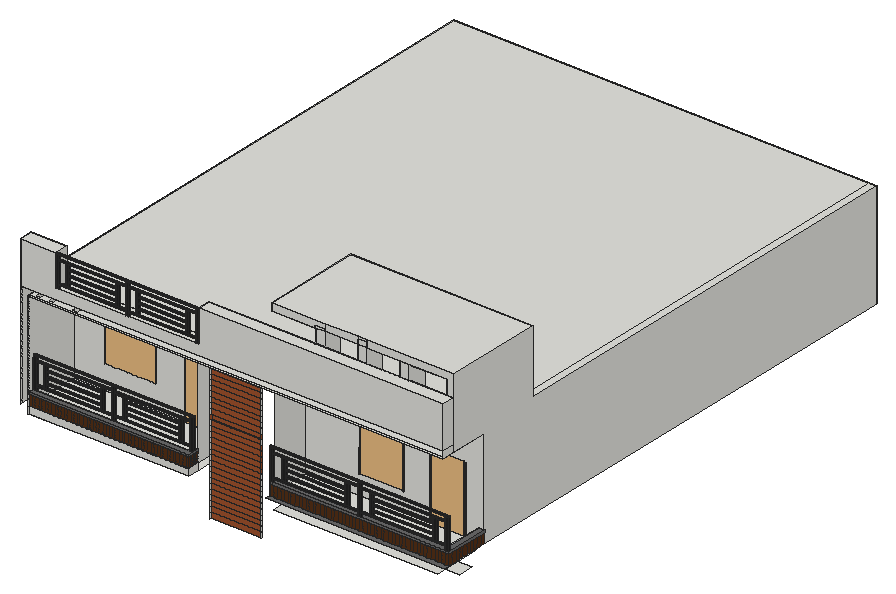
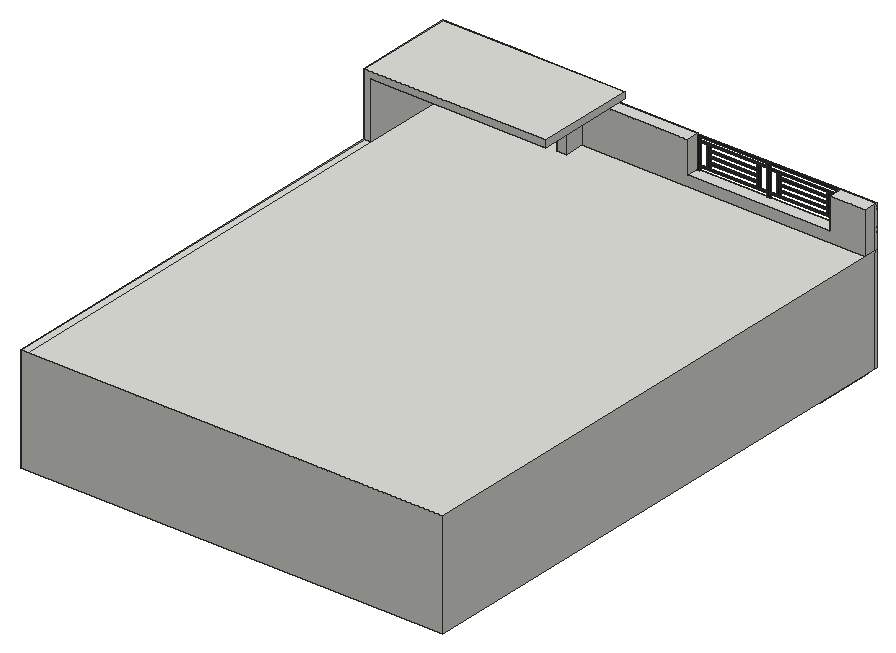
# SketchUp Ruby script. Lengths in inches.
U = 1.inch
M = Sketchup.active_model
def pt(a) = Geom::Point3d.new(a.map { |v| v * U })
def face(e, loops, mat)
  f = e.add_face(loops[0].map { |a| pt(a) })
  loops[1..].each { |l| e.add_face(l.map { |a| pt(a) }).erase! }
  f.material = f.back_material = mat if mat
  f
end
# faces: each face lists its corners as indices into pts; further lists are holes
def faces(e, pts, list, mat = nil) = list.each { |f| face(e, (f[0].is_a?(Array) ? f : [f]).map { |l| l.map { |i| pts[i] } }, mat) }
# xy, xz, yz: faces in a plane at the given z, y or x. An outline is a flat list of corners, or four numbers for a rectangle; further outlines are holes
def ring(l) = l.size == 4 ? [[l[0], l[1]], [l[2], l[1]], [l[2], l[3]], [l[0], l[3]]] : l.each_slice(2).to_a
def flat(e, list, mat, &to3) = list.each { |f| face(e, (f[0].is_a?(Array) ? f : [f]).map { |l| ring(l).map { |u, v| to3.(u, v) } }, mat) }
def xy(e, z, list, mat = nil) = flat(e, list, mat) { |x, y| [x, y, z] }
def xz(e, y, list, mat = nil) = flat(e, list, mat) { |x, z| [x, y, z] }
def yz(e, x, list, mat = nil) = flat(e, list, mat) { |y, z| [x, y, z] }
def lines(e, pts, list) = list.each { |a, b| e.add_line(pt(pts[a]), pt(pts[b])) }
# prism: a flat outline (further loops are holes) pulled along v
def prism(e, loops, v, mat = nil)
  f = face(e, loops, mat); d = Geom::Vector3d.new(v.map { |x| x * U })
  f.pushpull(f.normal.samedirection?(d) ? d.length : -d.length)
end
def box(e, o, s, mat = nil) = prism(e, [[o, [o[0] + s[0], o[1], o[2]], [o[0] + s[0], o[1] + s[1], o[2]], [o[0], o[1] + s[1], o[2]]]], [0, 0, s[2]], mat)
def at(x, y, z, deg = 0) = Geom::Transformation.translation(pt([x, y, z])) * Geom::Transformation.rotation(ORIGIN, Z_AXIS, deg.degrees)
def axes(o, x, y, z) = Geom::Transformation.new([*x, 0, *y, 0, *z, 0, *pt(o).to_a, 1])
def part(name) = M.definitions.add(name)
# library, detail: a bought-in or finely detailed component or shape, given as its bounding box
def library(name, o, s) = part(name).tap { |d| box(d.entities, o, s) }
def detail(e, o, s) = box(e.add_group.entities, o, s)
def put(e, d, t, mat = nil) = e.add_instance(d, t).tap { |i| i.material = mat if mat }
def group(e, t, mat = nil) = e.add_group.tap { |g| g.transformation = t; g.material = mat if mat }.entities
root = M.entities
M.materials.add("Painted Metal Railing").color = [35, 35, 35]
M.materials.add("[0042_Sienna]").color = [160, 82, 45]
M.materials.add("[0134_DimGray]").color = [105, 105, 105]
M.materials.add("[Wood Cherry Original]").color = [86, 49, 23]
c1 = library("PINTU 6 YA",[0,-0.6875,0],[35.83,8.07,80.71])
c2 = part("Post")
box(c2.entities,[-0.75,-0.75,0],[1.5,1.5,34.5],"Painted Metal Railing")
c3 = part("Group43\#1")
box(c3.entities,[-0.75,0,0],[1.5,73.5,1.5],"Painted Metal Railing")
c4 = part("Group46\#2")
box(c4.entities,[-0.75,0.75,0],[1.5,34.5,1.5],"Painted Metal Railing")
c5 = part("Group49\#1")
box(c5.entities,[-0.75,0.75,0],[1.5,34.5,1.5],"Painted Metal Railing")
c6 = part("Group52\#1")
box(c6.entities,[-0.75,0.75,0],[1.5,34.5,1.5],"Painted Metal Railing")
c7 = part("Group55\#1")
box(c7.entities,[-0.75,0.75,0],[1.5,34.5,1.5],"Painted Metal Railing")
c8 = part("Inner Post")
box(c8.entities,[-0.75,-0.75,0],[1.5,1.5,23.5],"Painted Metal Railing")
c9 = part("Group59\#1")
box(c9.entities,[-0.75,0.75,0],[1.5,24.5,1.5],"Painted Metal Railing")
c10 = part("Group62\#1")
box(c10.entities,[-0.75,0.75,0],[1.5,24.5,1.5],"Painted Metal Railing")
c11 = part("Group65\#1")
box(c11.entities,[-0.75,0.75,0],[1.5,24.5,1.5],"Painted Metal Railing")
c12 = part("Inner Posts and Rails\#2")
put(c12.entities,c8,at(0,0,0,90))
put(c12.entities,c8,at(0,26,0,90))
put(c12.entities,c9,at(0,0,4.75))
put(c12.entities,c10,at(0,0,11))
put(c12.entities,c11,at(0,0,17.25))
c13 = part("Group69\#1")
box(c13.entities,[-0.75,0.75,0],[1.5,24.5,1.5],"Painted Metal Railing")
c14 = part("Group72\#1")
box(c14.entities,[-0.75,0.75,0],[1.5,24.5,1.5],"Painted Metal Railing")
c15 = part("Group75\#1")
box(c15.entities,[-0.75,0.75,0],[1.5,24.5,1.5],"Painted Metal Railing")
c16 = part("Inner Posts and Rails\#3")
put(c16.entities,c8,at(0,0,0,90))
put(c16.entities,c8,at(0,26,0,90))
put(c16.entities,c13,at(0,0,4.75))
put(c16.entities,c14,at(0,0,11))
put(c16.entities,c15,at(0,0,17.25))
c17 = part("Railing Assembly 14\#1")
put(c17.entities,c2,at(0,0,0))
put(c17.entities,c2,at(36,0,0))
put(c17.entities,c2,at(72,0,0))
put(c17.entities,c3,at(-0.75,0,34.5,-90))
put(c17.entities,c4,at(0,0,4,-90))
put(c17.entities,c5,at(36,0,4,-90))
put(c17.entities,c6,at(0,0,29,-90))
put(c17.entities,c7,at(36,0,29,-90))
put(c17.entities,c12,at(5,0,5.5,-90))
put(c17.entities,c16,at(41,0,5.5,-90))
c18 = library("Group\#6",[0,0,0],[8.07,62.0625,54])
xy(root,321.9375,[[415.76,55.8125,455.32,73]])
xy(root,323.32,[[334.19,55.8125,396.26,70.4375]])
xy(root,332.51,[[33.6,70.1875,103.97,80.1875]])
xy(root,335.1875,[[131.125,70.1875,180.3125,90.9375]])
xy(root,352,[[8,2.66,8,70.1875,189.625,70.1875,189.625,15.9375,190.03,15.9375,190.03,2.66],[286.5625,3.0625,472.04,55.8125]])
xy(root,360,[[8,2.66,190.03,2.66,190.03,15.9375,189.625,15.9375,189.625,3.0625,8,3.0625],[8,3.0625,8,9.0625,183.625,9.0625,183.625,15.9375,189.625,15.9375,189.625,3.0625],[8,9.0625,183.625,9.0625,183.625,15.9375,189.625,15.9375,189.625,66.3125,182.5,66.3125,182.5,77.1875,134.19,77.1875,134.19,66.3125,8,66.3125],[276.8125,9.0625,276.8125,15.9375,474,15.9375,474,59.375,480,59.375,480,9.0625],[276.8125,15.9375,474,15.9375,474,59.375,457.04,59.375,457.04,75.5,418.72,75.5,418.72,59.375,276.8125,59.375]])
xy(root,360,[[276.8125,3.0625,480,9.0625]],"[0134_DimGray]")
xy(root,372,[[8,2.66,190.03,3.0625],[8,3.0625,8,9.0625,183.625,9.0625,183.625,15.9375,189.625,15.9375,189.625,3.0625],[189.625,3.0625,190.03,15.9375],[276.8125,8.66,480.4,9.0625],[276.8125,9.0625,276.8125,15.9375,474,15.9375,474,59.375,480,59.375,480,9.0625],
  [480,9.0625,480.4,59.375]])
xy(root,374,[[8,2.66,190.03,2.66,190.03,15.9375,183.625,15.9375,183.625,9.0625,8,9.0625]],"[0134_DimGray]")
xy(root,374.875,[[276.8125,8.66,480.4,8.66,480.4,59.375,474,59.375,474,15.9375,276.8125,15.9375]],"[0134_DimGray]")
xy(root,381.34,[[338.1875,59.375,387.9375,69.0625]])
xy(root,387.125,[[44.07,66.3125,101.07,89.625]])
xy(root,407.98,[[203.35,17.0625,260.98,18.1875]],"[0042_Sienna]")
xy(root,413.85,[[203.35,17.0625,260.98,18.1875]])
xy(root,436.06,[[338.28,59.375,388.03,69.0625]])
xy(root,436.3125,[[418.72,59.375,457.04,75.5]])
xy(root,440.4375,[[44.07,66.3125,101.07,89.625]])
xy(root,446.5625,[[134.19,66.3125,182.5,77.1875]])
xy(root,460.87,[[203.35,15.54,260.98,17.0625]])
xy(root,466.75,[[203.35,15.54,260.98,17.0625]],"[0042_Sienna]")
xy(root,471.9375,[[41.12,5.07,47.93,11.88]])
xy(root,472.625,[[8,1,480,3.0625],[[8,3.0625,8,66.3125,189.625,66.3125,189.625,15.9375,203.35,15.9375,203.35,17.0625,260.98,17.0625,260.98,15.9375,276.8125,15.9375,276.8125,59.375,480,59.375,480,3.0625],[13.71,5.07,20.52,11.88],[27.41,5.07,34.23,11.88],[54.83,5.07,61.64,11.88]]])
xy(root,480,[[0,1,480,15.9375],[0,15.9375,322.54,15.9375,322.54,37.75,333.36,37.75,333.36,15.9375,370.7,15.9375,370.7,37.75,381.51,37.75,381.51,15.9375,418.86,15.9375,418.86,37.75,429.67,37.75,429.67,15.9375,472,15.9375,472,615.9375,0,615.9375],[472,128.18,480,615.9375]])
xy(root,491.72,[[40.47,1,202.15,15.9375]])
xy(root,528,[[0,1,40.47,15.9375],[202.15,1,480,15.9375],[322.54,15.9375,333.36,17.25]])
xy(root,544,[[273.3125,15.9375,273.3125,128.18,472,128.18,472,15.9375,429.67,15.9375,429.67,37.75,418.86,37.75,418.86,15.9375,333.36,15.9375,333.36,17.25,322.54,17.25,322.54,15.9375],[322.54,15.9375,333.36,17.25]])
xy(root,546.3125,[[322.54,15.9375,333.36,37.75]])
xy(root,549.9375,[[370.7,15.9375,381.51,37.75]])
xy(root,552,[[273.3125,15.9375,480,128.18]])
xz(root,1,[[0,480,480,480,480,528,202.15,528,202.15,491.72,40.47,491.72,40.47,528,0,528]])
xz(root,2.66,[[8,352,190.03,360]])
xz(root,2.66,[[8,372,190.03,374]],"[0134_DimGray]")
xz(root,3.0625,[[8,360,11.63,372],[11.63,360,15.27,372],[15.27,360,18.9,372],[18.9,360,22.53,372],[22.53,360,26.16,372],
  [26.16,360,29.8,372],[29.8,360,33.43,372],[33.43,360,37.06,372],[37.06,360,40.69,372],[40.69,360,44.33,372],
  [44.33,360,47.96,372],[47.96,360,51.59,372],[51.59,360,55.22,372],[55.22,360,58.86,372],[58.86,360,62.49,372],
  [62.49,360,66.12,372],[66.12,360,69.75,372],[69.75,360,73.38,372],[73.38,360,77.02,372],[77.02,360,80.65,372],
  [80.65,360,84.28,372],[84.28,360,87.91,372],[87.91,360,91.55,372],[91.55,360,95.18,372],[95.18,360,98.8125,372],
  [98.8125,360,102.44,372],[102.44,360,106.08,372],[106.08,360,109.71,372],[109.71,360,113.34,372],[113.34,360,116.97,372],
  [116.97,360,120.61,372],[120.61,360,124.24,372],[124.24,360,127.87,372],[127.87,360,131.5,372],[131.5,360,135.14,372],
  [135.14,360,138.77,372],[138.77,360,142.4,372],[142.4,360,146.03,372],[146.03,360,149.67,372],[149.67,360,153.3,372],
  [153.3,360,156.93,372],[156.93,360,160.56,372],[160.56,360,164.2,372],[164.2,360,167.83,372],[167.83,360,171.46,372],
  [171.46,360,175.09,372],[175.09,360,178.73,372],[178.73,360,182.36,372],[182.36,360,185.99,372],[185.99,360,189.625,372]],"[Wood Cherry Original]")
xz(root,8.66,[[276.8125,372,480.4,374.875]],"[0134_DimGray]")
xz(root,9.0625,[[8,360,183.625,372],[8,372,183.625,374]])
xz(root,9.0625,[[276.8125,360,280.875,372],[280.875,360,284.94,372],[284.94,360,289,372],[289,360,293.07,372],[293.07,360,297.13,372],
  [297.13,360,301.19,372],[301.19,360,305.26,372],[305.26,360,309.32,372],[309.32,360,313.39,372],[313.39,360,317.45,372],
  [317.45,360,321.51,372],[321.51,360,325.58,372],[325.58,360,329.64,372],[329.64,360,333.7,372],[333.7,360,337.77,372],
  [337.77,360,341.83,372],[341.83,360,345.9,372],[345.9,360,349.96,372],[349.96,360,354.02,372],[354.02,360,358.09,372],
  [358.09,360,362.15,372],[362.15,360,366.21,372],[366.21,360,370.28,372],[370.28,360,374.34,372],[374.34,360,378.41,372],
  [378.41,360,382.47,372],[382.47,360,386.53,372],[386.53,360,390.6,372],[390.6,360,394.66,372],[394.66,360,398.72,372],
  [398.72,360,402.79,372],[402.79,360,406.85,372],[406.85,360,410.92,372],[410.92,360,414.98,372],[414.98,360,419.04,372],
  [419.04,360,423.11,372],[423.11,360,427.17,372],[427.17,360,431.23,372],[431.23,360,435.3,372],[435.3,360,439.36,372],
  [439.36,360,443.43,372],[443.43,360,447.49,372],[447.49,360,451.55,372],[451.55,360,455.62,372],[455.62,360,459.68,372],
  [459.68,360,463.74,372],[463.74,360,467.81,372],[467.81,360,471.87,372],[471.87,360,475.9375,372],[475.9375,360,480,372]],"[Wood Cherry Original]")
xz(root,15.54,[[203.35,460.87,260.98,466.75]],"[0042_Sienna]")
xz(root,15.9375,[[183.625,360,189.625,372],[276.8125,360,474,372],[183.625,372,189.625,374],[189.625,372,190.03,374],[276.8125,372,474,374.875],
  [0,480,0,528,40.47,528,40.47,491.72,202.15,491.72,202.15,528,322.54,528,322.54,480],[322.54,480,333.36,528],[333.36,480,370.7,528],[370.7,480,381.51,528],[381.51,480,418.86,528],
  [418.86,480,429.67,528],[429.67,480,472,528],[472,480,480,528],[370.7,528,381.51,544],[472,528,480,528,480,552,381.51,552,381.51,544,472,544],
  [418.86,528,429.67,544],[273.3125,544,322.54,544,322.54,546.3125,333.36,546.3125,333.36,552,273.3125,552],[322.54,544,333.36,546.3125],[333.36,544,370.7,552],[370.7,544,381.51,549.9375],
  [370.7,549.9375,381.51,552]])
xz(root,17.0625,[[203.35,308.07,260.98,313.94],[203.35,313.94,260.98,319.82],[203.35,319.82,260.98,325.7],[203.35,325.7,260.98,331.57],[203.35,331.57,260.98,337.45],
  [203.35,337.45,260.98,343.33],[203.35,343.33,260.98,349.21],[203.35,349.21,260.98,355.08],[203.35,355.08,260.98,360.96],[203.35,360.96,260.98,366.84],
  [203.35,366.84,260.98,372.71],[203.35,372.71,260.98,378.59],[203.35,378.59,260.98,384.47],[203.35,384.47,260.98,390.35],[203.35,390.35,260.98,396.22],
  [203.35,396.22,260.98,402.1],[203.35,402.1,260.98,407.98],[203.35,413.85,260.98,419.73],[203.35,419.73,260.98,425.61],[203.35,425.61,260.98,431.49],
  [203.35,431.49,260.98,437.36],[203.35,437.36,260.98,443.24],[203.35,443.24,260.98,449.12],[203.35,449.12,260.98,454.99],[203.35,454.99,260.98,460.87],
  [203.35,466.75,260.98,472.625]],"[0042_Sienna]")
xz(root,17.25,[[322.54,528,333.36,544]])
xz(root,18.1875,[[203.35,407.98,260.98,413.85]],"[0042_Sienna]")
xz(root,37.75,[[322.54,480,333.36,546.3125],[370.7,480,381.51,549.9375],[418.86,480,429.67,544]])
xz(root,59.375,[[[276.8125,360,418.72,360,418.72,436.3125,457.04,436.3125,457.04,360,474,360,474,374.875,480,374.875,480,472.625,276.8125,472.625],[338.1875,381.34,338.28,436.06,388.03,436.06,387.9375,381.34]],[474,360,480,372],[474,372,480,374.875],[480,372,480.4,374.875]])
xz(root,66.3125,[[[8,360,134.19,360,134.19,446.5625,182.5,446.5625,182.5,360,189.625,360,189.625,472.625,8,472.625],[44.07,387.125,101.07,440.4375]]])
xz(root,69.0625,[[338.1875,381.34,387.9375,381.34,388.03,436.06,338.28,436.06]])
xz(root,75.5,[[418.72,360,457.04,436.3125]])
xz(root,77.1875,[[134.19,360,182.5,446.5625]])
xz(root,89.625,[[44.07,387.125,101.07,440.4375]])
xz(root,128.18,[[472,480,472,544,273.3125,544,273.3125,552,480,552,480,480]])
xz(root,615.9375,[[0,360,480,480]])
yz(root,0,[[1,360,3.0625,480],[3.0625,360,615.9375,480],[1,480,3.0625,528],[3.0625,480,15.9375,528]])
yz(root,8,[[1,352,2.66,360],[1,360,3.0625,360,3.0625,372,2.66,372,2.66,374,3.0625,374,3.0625,472.625,1,472.625],[3.0625,360,9.0625,372],[9.0625,360,66.3125,360,66.3125,472.625,3.0625,472.625,3.0625,374,9.0625,374],[2.66,372,9.0625,374]])
yz(root,40.47,[[1,491.72,15.9375,528]])
yz(root,44.07,[[66.3125,387.125,89.625,440.4375]])
yz(root,101.07,[[66.3125,387.125,89.625,440.4375]])
yz(root,134.19,[[66.3125,360,77.1875,446.5625]])
yz(root,182.5,[[66.3125,360,77.1875,446.5625]])
yz(root,183.625,[[9.0625,360,15.9375,372],[9.0625,372,15.9375,374]])
yz(root,189.625,[[15.9375,360,66.3125,472.625]])
yz(root,189.625,[[3.0625,360,4.9,372],[4.9,360,6.74,372],[6.74,360,8.58,372],[8.58,360,10.42,372],[10.42,360,12.26,372],
  [12.26,360,14.1,372],[14.1,360,15.9375,372]],"[Wood Cherry Original]")
yz(root,190.03,[[2.66,352,15.9375,360]])
yz(root,190.03,[[2.66,372,15.9375,374]],"[0134_DimGray]")
yz(root,202.15,[[1,491.72,15.9375,528]])
yz(root,203.35,[[15.9375,308.07,17.0625,313.94],[15.9375,313.94,17.0625,319.82],[15.9375,319.82,17.0625,325.7],[15.9375,325.7,17.0625,331.57],[15.9375,331.57,17.0625,337.45],
  [15.9375,337.45,17.0625,343.33],[15.9375,343.33,17.0625,349.21],[15.9375,349.21,17.0625,355.08],[15.9375,355.08,17.0625,360.96],[15.9375,360.96,17.0625,366.84],
  [15.9375,366.84,17.0625,372.71],[15.9375,372.71,17.0625,378.59],[15.9375,378.59,17.0625,384.47],[15.9375,384.47,17.0625,390.35],[15.9375,390.35,17.0625,396.22],
  [15.9375,396.22,17.0625,402.1],[15.9375,402.1,17.0625,407.98],[15.9375,413.85,17.0625,419.73],[15.9375,419.73,17.0625,425.61],[15.9375,425.61,17.0625,431.49],
  [15.9375,431.49,17.0625,437.36],[15.9375,437.36,17.0625,443.24],[15.9375,443.24,17.0625,449.12],[15.9375,449.12,17.0625,454.99],[15.9375,454.99,17.0625,460.87],
  [15.9375,466.75,17.0625,472.625]])
yz(root,203.35,[[15.9375,407.98,18.1875,413.85],[15.54,460.87,15.9375,466.75]],"[0042_Sienna]")
yz(root,260.98,[[15.9375,308.07,17.0625,313.94],[15.9375,313.94,17.0625,319.82],[15.9375,319.82,17.0625,325.7],[15.9375,325.7,17.0625,331.57],[15.9375,331.57,17.0625,337.45],
  [15.9375,337.45,17.0625,343.33],[15.9375,343.33,17.0625,349.21],[15.9375,349.21,17.0625,355.08],[15.9375,355.08,17.0625,360.96],[15.9375,360.96,17.0625,366.84],
  [15.9375,366.84,17.0625,372.71],[15.9375,402.1,17.0625,407.98],[15.9375,413.85,17.0625,419.73],[15.9375,419.73,17.0625,425.61],[15.9375,425.61,17.0625,431.49],
  [15.9375,431.49,17.0625,437.36],[15.9375,437.36,17.0625,443.24],[15.9375,443.24,17.0625,449.12],[15.9375,449.12,17.0625,454.99],[15.9375,454.99,17.0625,460.87],
  [15.54,460.87,15.9375,466.75],[15.9375,466.75,17.0625,472.625]])
yz(root,260.98,[[15.9375,372.71,17.0625,378.59],[15.9375,378.59,17.0625,384.47],[15.9375,384.47,17.0625,390.35],[15.9375,390.35,17.0625,396.22],[15.9375,396.22,17.0625,402.1],
  [15.9375,407.98,18.1875,413.85]],"[0042_Sienna]")
yz(root,273.3125,[[15.9375,544,128.18,552]])
yz(root,276.8125,[[9.0625,360,15.9375,372],[15.9375,360,59.375,472.625]])
yz(root,276.8125,[[8.66,372,15.9375,374.875]],"[0134_DimGray]")
yz(root,322.54,[[15.9375,480,15.9375,528,17.25,528,17.25,544,15.9375,544,15.9375,546.3125,37.75,546.3125,37.75,480]])
yz(root,333.36,[[15.9375,480,37.75,480,37.75,546.3125,15.9375,546.3125,15.9375,544,17.25,544,17.25,528,15.9375,528]])
yz(root,370.7,[[15.9375,480,37.75,549.9375]])
yz(root,381.51,[[15.9375,480,37.75,549.9375]])
yz(root,418.72,[[59.375,360,75.5,436.3125]])
yz(root,418.86,[[15.9375,480,37.75,544]])
yz(root,429.67,[[15.9375,480,37.75,544]])
yz(root,457.04,[[59.375,360,75.5,436.3125]])
yz(root,472,[[15.9375,480,128.18,544]])
yz(root,474,[[15.9375,360,59.375,372],[15.9375,372,59.375,374.875]])
yz(root,480,[[59.375,360,615.9375,360,615.9375,480,128.18,480,128.18,552,15.9375,552,15.9375,472.625,59.375,472.625],[1,472.625,15.9375,480],[1,480,15.9375,528]])
yz(root,480,[[9.0625,360,14.09,372],[14.09,360,19.125,372],[19.125,360,24.16,372],[24.16,360,29.1875,372],[29.1875,360,34.22,372],
  [34.22,360,39.25,372],[39.25,360,44.28,372],[44.28,360,49.3125,372],[49.3125,360,54.34,372],[54.34,360,59.375,372]],"[Wood Cherry Original]")
yz(root,480.4,[[8.66,372,59.375,374.875]],"[0134_DimGray]")
p = [[338.28,59.375,436.06],[338.1875,59.375,381.34],[338.1875,69.0625,381.34],[338.28,69.0625,436.06],[387.9375,59.375,381.34],[388.03,59.375,436.06],
  [388.03,69.0625,436.06],[387.9375,69.0625,381.34]]
faces(root,p,[[0,1,2,3],[4,5,6,7]])
put(root,c1,axes([134.24,66.3125,360],[1.3471,0,0],[0,0.5,0],[0,0,1.07253]))
put(root,c1,axes([419.22,59.69,360],[1.10418,0,0],[0,0.45732,0],[0,0,0.94553]))
put(root,c17,axes([9.86,9.8125,374],[2.47653,0,0],[0,1,0],[0,0,1]))
put(root,c17,axes([278.96,9.41,374.875],[2.7689,0,0],[0,1,0],[0,0,1]))
put(root,c18,axes([388.67,59.375,381.34],[0,0.78,0],[-0.8112,0,0],[0,0,1.0062]))
put(root,c18,axes([101.07,66.3125,387.125],[0,1,0],[-0.91843,0,0],[0,0,0.98727]))
put(root,c17,axes([42.12,1.75,491.72],[2.19983,0,0],[0,1,0],[0,0,1]))
